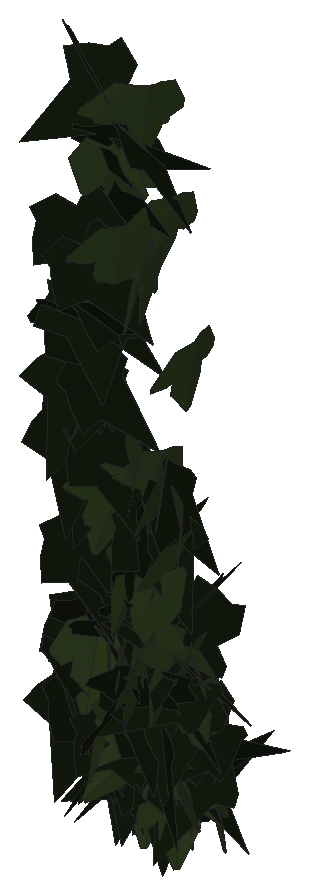
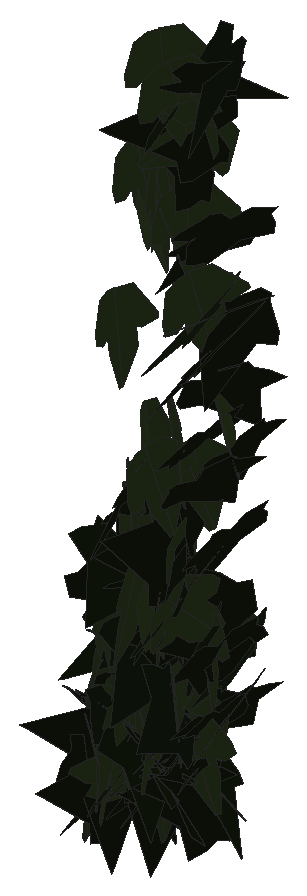
# SketchUp Ruby script. Lengths in inches.
U = 1.inch
M = Sketchup.active_model
def pt(a) = Geom::Point3d.new(a.map { |v| v * U })
def face(e, loops, mat)
  f = e.add_face(loops[0].map { |a| pt(a) })
  loops[1..].each { |l| e.add_face(l.map { |a| pt(a) }).erase! }
  f.material = f.back_material = mat if mat
  f
end
# faces: each face lists its corners as indices into pts; further lists are holes
def faces(e, pts, list, mat = nil) = list.each { |f| face(e, (f[0].is_a?(Array) ? f : [f]).map { |l| l.map { |i| pts[i] } }, mat) }
# xy, xz, yz: faces in a plane at the given z, y or x. An outline is a flat list of corners, or four numbers for a rectangle; further outlines are holes
def ring(l) = l.size == 4 ? [[l[0], l[1]], [l[2], l[1]], [l[2], l[3]], [l[0], l[3]]] : l.each_slice(2).to_a
def flat(e, list, mat, &to3) = list.each { |f| face(e, (f[0].is_a?(Array) ? f : [f]).map { |l| ring(l).map { |u, v| to3.(u, v) } }, mat) }
def xy(e, z, list, mat = nil) = flat(e, list, mat) { |x, y| [x, y, z] }
def xz(e, y, list, mat = nil) = flat(e, list, mat) { |x, z| [x, y, z] }
def yz(e, x, list, mat = nil) = flat(e, list, mat) { |y, z| [x, y, z] }
def lines(e, pts, list) = list.each { |a, b| e.add_line(pt(pts[a]), pt(pts[b])) }
# prism: a flat outline (further loops are holes) pulled along v
def prism(e, loops, v, mat = nil)
  f = face(e, loops, mat); d = Geom::Vector3d.new(v.map { |x| x * U })
  f.pushpull(f.normal.samedirection?(d) ? d.length : -d.length)
end
def box(e, o, s, mat = nil) = prism(e, [[o, [o[0] + s[0], o[1], o[2]], [o[0] + s[0], o[1] + s[1], o[2]], [o[0], o[1] + s[1], o[2]]]], [0, 0, s[2]], mat)
def at(x, y, z, deg = 0) = Geom::Transformation.translation(pt([x, y, z])) * Geom::Transformation.rotation(ORIGIN, Z_AXIS, deg.degrees)
def axes(o, x, y, z) = Geom::Transformation.new([*x, 0, *y, 0, *z, 0, *pt(o).to_a, 1])
def part(name) = M.definitions.add(name)
# library, detail: a bought-in or finely detailed component or shape, given as its bounding box
def library(name, o, s) = part(name).tap { |d| box(d.entities, o, s) }
def detail(e, o, s) = box(e.add_group.entities, o, s)
def put(e, d, t, mat = nil) = e.add_instance(d, t).tap { |i| i.material = mat if mat }
def group(e, t, mat = nil) = e.add_group.tap { |g| g.transformation = t; g.material = mat if mat }.entities
root = M.entities
M.materials.add("efeu1").color = [18, 25, 13]
M.materials.add("efeu2").color = [43, 57, 29]
c1 = part("ivyleaf_9")
p = [[1.54,2.16,1.25],[1.36,2.04,1.19],[-0.21,0.99,0.68],[-0.71,1.11,0.82],[-0.85,0.86,0.67],[-0.8,0.17,0.21],
  [-0.9,-0.01,0.1],[-0.67,-0.16,-0.02],[-0.08,-0.08,-0.05],[-0.03,-0.6,-0.4],[0.65,-0.88,-0.66],[0.83,-0.6,-0.49],
  [1.29,-0.42,-0.43],[1.8125,-0.07,-0.26],[1.21,0.44,0.15]]
faces(c1.entities,p,[[0,1,2,3,4,5,6,7,8,9,10,11,12,13,14]],"efeu1")
c2 = part("ivyleaf_10")
p = [[0,0.5,-0.03],[-0.0625,2.02,-0.43],[-0.19,2.01,-0.46],[-0.54,1.05,-0.29],[-0.52,0.625,-0.18],[-0.83,0.76,-0.28],
  [-1.16,0.64,-0.33],[-1.15,0.33,-0.24],[-0.77,-0.39,0.02],[-0.3,-0.51,0.16],[0.04,-0.48,0.23],[-0.02,2.01,-0.4375],
  [-0.06,2.01,-0.43],[0.04,-0.49,0.23],[0.67,-0.49,0.14],[1.38,0.36,-0.2],[1.375,0.51,-0.24],[0.81,0.65,-0.19],
  [0.62,0.59,-0.15],[0.6,1.09,-0.28],[0.5,1.23,-0.31]]
faces(c2.entities,p,[[0,1,2,3,4,5,6,7,8,9,10],[11,12,0,13,14,15,16,17,18,19,20]],"efeu2")
put(root,c1,axes([24.9,223.875,227.96],[-0.03734,-0.49581,0.05269],[-0.00909,-0.05215,-0.49719],[0.49852,-0.03809,-0.00512]))
put(root,c2,axes([25.2,224.25,223.83],[0.42311,-0.0185,-0.26577],[-0.23449,0.21088,-0.388],[0.12645,0.45297,0.16978]))
put(root,c1,axes([24.92,224.1,225.18],[0.01701,-0.48645,-0.11436],[-0.01724,0.11378,-0.48658],[0.49941,0.0205,-0.0129]))
put(root,c2,axes([25.09,223.83,228.52],[0.27311,-0.41851,0.01623],[0.00957,-0.01314,-0.49974],[0.41871,0.27328,0.00084]))
put(root,c1,axes([25.11,223.47,229.91],[0.3697,0.30061,-0.15152],[-0.13618,-0.07226,-0.47564],[-0.30786,0.39295,0.02845]))
put(root,c1,axes([24.91,223.53,224.96],[0.39664,-0.25422,-0.16747],[-0.09197,0.16213,-0.46396],[0.2902,0.39885,0.08185]))
put(root,c1,axes([24.92,223.74,224.14],[0.259,-0.41597,-0.09944],[-0.05405,0.08349,-0.49001],[0.42426,0.26458,-0.00172]))
put(root,c1,axes([25.13,223.63,233.63],[0.38485,-0.02875,-0.31791],[-0.3081,0.09677,-0.38172],[0.08348,0.4897,0.05677]))
put(root,c1,axes([25.16,223.85,228.86],[-0.29876,-0.4009,-0.00486],[0.00283,0.00395,-0.49998],[0.40092,-0.29877,-0.00009]))
put(root,c1,axes([25.07,224.11,222.95],[-0.05747,0.40596,-0.28617],[-0.06168,0.28001,0.40962],[0.49284,0.08239,0.0179]))
put(root,c1,axes([25.24,224.52,224.32],[0.07525,0.25877,0.42116],[0.02834,0.42306,-0.26499],[-0.49349,0.06375,0.049]))
put(root,c1,axes([24.93,224.39,224.26],[0.18953,-0.41983,-0.19448],[0.00009,0.2102,-0.45367],[0.46269,0.17194,0.07975]))
put(root,c1,axes([25.1,224.25,227.63],[-0.18158,-0.46064,0.06957],[0.00543,-0.07676,-0.49404],[0.46583,-0.17867,0.03288]))
put(root,c1,axes([25.08,223.86,224.08],[-0.14703,-0.46431,0.11314],[0.00838,-0.12086,-0.4851],[0.47782,-0.14075,0.04332]))
put(root,c2,axes([25.19,224.61,224.72],[0.23477,-0.41994,-0.13614],[-0.01582,0.1461,-0.47792],[0.44117,0.22871,0.05531]))
put(root,c1,axes([24.96,224.06,224.15],[0.18569,-0.40449,-0.22783],[-0.03218,0.23357,-0.44092],[0.46312,0.17841,0.06071]))
put(root,c1,axes([25.41,223.72,223.3],[-0.22871,0.44254,0.04299],[-0.01825,0.03896,-0.49815],[-0.44425,-0.22944,-0.00167]))
put(root,c1,axes([24.98,223.8,229.56],[0.17395,-0.46805,-0.02591],[0.02253,0.03595,-0.4982],[0.46822,0.17216,0.03359]))
put(root,c1,axes([25.02,223.74,231.22],[0.01891,-0.42163,-0.26809],[0.08632,0.267,-0.41383],[0.49213,-0.03063,0.08288]))
put(root,c2,axes([25.34,224.39,225.77],[0.14772,0.32658,-0.3486],[-0.20913,-0.28385,-0.35454],[-0.42947,0.25054,0.05274]))
put(root,c2,axes([25.31,223.83,225.2],[0.37751,-0.25512,-0.20592],[-0.08376,0.22856,-0.43674],[0.31697,0.36424,0.12983]))
put(root,c1,axes([25.11,223.63,226.6],[0.12625,-0.45515,-0.164],[-0.03084,0.16158,-0.47217],[0.48282,0.12933,0.01273]))
put(root,c1,axes([25.01,223.66,225.25],[0.32737,0.08964,0.36714],[0.34482,0.12797,-0.33871],[-0.15469,0.47496,0.02196]))
put(root,c2,axes([25.42,223.95,230.14],[-0.20271,-0.43927,0.12631],[-0.00107,-0.13771,-0.48066],[0.45706,-0.19514,0.05489]))
put(root,c1,axes([25.31,224.64,223.375],[-0.23606,-0.43533,-0.069],[0.04063,0.05645,-0.49514],[0.43889,-0.23938,0.00872]))
put(root,c1,axes([25.14,223.875,229.85],[-0.05658,-0.49678,0.00185],[0.1772,-0.02192,-0.46703],[0.46411,-0.0522,0.17854]))
put(root,c1,axes([25.6,223.9,233.13],[-0.39215,-0.1953,0.24099],[-0.18845,-0.15856,-0.43514],[0.2464,-0.4321,0.05075]))
put(root,c1,axes([25.16,223.87,229.99],[0.36504,-0.2859,-0.1871],[-0.06885,0.20663,-0.45007],[0.33467,0.35435,0.11149]))
put(root,c1,axes([25.13,224.14,223.58],[0.26347,-0.42121,0.05626],[0.02025,-0.05368,-0.4967],[0.42447,0.26401,-0.01123]))
put(root,c2,axes([25.41,223.625,225.24],[0.37271,0.32855,-0.05611],[-0.04662,-0.03196,-0.49679],[-0.33003,0.37555,0.00681]))
put(root,c1,axes([25.85,224.3125,222.99],[-0.20139,0.018,-0.45729],[-0.45662,-0.04133,0.19947],[-0.03062,0.49796,0.03309]))
put(root,c2,axes([25.5,224.51,223.46],[0.01115,-0.49259,-0.08504],[0.01777,0.0854,-0.49233],[0.49956,0.00796,0.01941]))
put(root,c1,axes([25.68,224.3,223.45],[-0.38287,0.25781,-0.19222],[0.09892,-0.18996,-0.45181],[-0.30598,-0.38399,0.09446]))
put(root,c2,axes([25.45,224.02,223.66],[-0.02991,-0.36564,-0.33972],[0.14889,0.3183,-0.35569],[0.47638,-0.12244,0.08984]))
put(root,c1,axes([25.3,224.12,226.02],[0.13597,-0.46864,0.10904],[0.03253,-0.1041,-0.48796],[0.48006,0.13979,0.00218]))
put(root,c1,axes([25.85,223.98,223.48],[-0.4524,0.1949,0.0857],[-0.08114,0.02825,-0.49256],[-0.19684,-0.45958,0.00606]))
put(root,c1,axes([25.45,224.46,223.46],[-0.11373,-0.48677,0.01121],[-0.00287,-0.01084,-0.49987],[0.48689,-0.11376,-0.00033]))
put(root,c1,axes([25.31,223.55,230.84],[0.14695,-0.3866,-0.28098],[0.0491,0.30462,-0.39344],[0.47539,0.08804,0.12748]))
put(root,c1,axes([25.78,224.52,223.6875],[-0.03757,0.48497,0.11574],[-0.07361,0.1094,-0.4823],[-0.49312,-0.05328,0.06318]))
put(root,c2,axes([25.6875,223.78,227.46],[-0.29374,-0.36021,0.18429],[-0.04949,-0.19404,-0.45815],[0.40158,-0.28739,0.07834]))
put(root,c2,axes([25.43,223.92,224.03],[-0.3174,-0.17678,-0.34352],[0.28878,0.18678,-0.36293],[0.25664,-0.42879,-0.01646]))
put(root,c2,axes([25.52,223.98,224.08],[0.07761,-0.32504,0.37192],[0.14468,-0.34501,-0.33171],[0.47227,0.15911,0.0405]))
put(root,c1,axes([25.39,223.47,229.16],[0.29346,-0.30224,-0.26932],[-0.07899,0.28349,-0.40422],[0.39704,0.27979,0.11864]))
put(root,c1,axes([25.38,223.8,228.01],[0.14786,-0.45519,-0.14471],[0.00546,0.15309,-0.47596],[0.47761,0.13917,0.05024]))
put(root,c1,axes([25.35,224.09,224.97],[0.09887,-0.34154,0.35153],[0.18408,-0.30648,-0.34955],[0.45425,0.19854,0.06514]))
put(root,c1,axes([25.73,224.26,223.29],[0.25444,0.39417,-0.17289],[-0.10681,-0.13673,-0.46893],[-0.41696,0.27556,0.01462]))
put(root,c1,axes([25.42,224.52,225.6875],[0.18051,-0.44663,0.13392],[0.06369,-0.11865,-0.48153],[0.46191,0.1909,0.01406]))
put(root,c1,axes([25.58,223.54,225.55],[0.3629,0.33503,0.07786],[0.06042,0.04933,-0.49388],[-0.33861,0.36786,-0.00468]))
put(root,c2,axes([25.77,223.76,225.33],[0.23914,-0.37135,-0.23432],[-0.04848,0.24286,-0.43436],[0.43642,0.23047,0.08015]))
put(root,c2,axes([25.8,223.64,231.13],[-0.22317,-0.44684,0.02305],[-0.00819,-0.02167,-0.49946],[0.44735,-0.22331,0.00235]))
put(root,c1,axes([25.82,223.28,224.31],[0.05577,0.40111,0.29326],[0.03897,0.29066,-0.40497],[-0.49535,0.06803,0.00115]))
put(root,c2,axes([25.52,223.58,232.38],[-0.21529,-0.20983,-0.39952],[0.36217,0.18374,-0.29167],[0.26922,-0.41498,0.07287]))
put(root,c1,axes([25.35,224.09,223.08],[0.34789,0.18804,-0.30596],[0.25695,0.16726,0.39497],[0.25089,-0.43205,0.01975]))
put(root,c2,axes([25.83,223.88,233.04],[-0.25752,-0.41224,0.11724],[-0.00377,-0.13459,-0.48153],[0.42857,-0.24889,0.06621]))
put(root,c1,axes([25.54,224.55,223.1875],[0.15715,-0.47347,0.03363],[0.00154,-0.03492,-0.49878],[0.47466,0.15687,-0.00951]))
put(root,c2,axes([25.85,224.29,227.59],[-0.08648,-0.47813,0.11795],[-0.00587,-0.11874,-0.48566],[0.49243,-0.08538,0.01493]))
put(root,c2,axes([25.83,224.48,223.51],[-0.21316,-0.43896,0.10898],[0.03655,-0.1368,-0.47953],[0.45081,-0.19647,0.09041]))
put(root,c2,axes([25.92,223.94,223.71],[-0.19839,-0.20561,0.41033],[-0.08658,-0.42223,-0.25343],[0.45072,-0.17161,0.13192]))
put(root,c1,axes([25.57,224.08,224],[0.32196,-0.36621,-0.1106],[-0.05263,0.10077,-0.4869],[0.37891,0.32517,0.02634]))
put(root,c1,axes([26.09,223.52,226.49],[-0.04756,0.06042,0.49405],[-0.21784,0.44372,-0.07524],[-0.44753,-0.22241,-0.01588]))
put(root,c1,axes([25.51,224.42,225.6],[0.09186,-0.22297,0.438],[0.18062,-0.39909,-0.24104],[0.4571,0.20251,0.00723]))
put(root,c1,axes([25.85,224.125,224.91],[0.22816,0.40693,0.17988],[-0.02422,0.21321,-0.45161],[-0.44425,0.19736,0.117]))
put(root,c2,axes([25.83,223.98,225.48],[0.1085,-0.45016,-0.18864],[0.03984,0.20077,-0.45619],[0.48646,0.08397,0.07944]))
put(root,c1,axes([25.43,223.59,232.34],[0.3556,-0.02951,0.35026],[0.35117,0.05138,-0.35219],[-0.01521,0.49648,0.05726]))
put(root,c2,axes([25.87,224.24,225.56],[0.08952,-0.48486,0.08304],[0.00652,-0.08323,-0.49298],[0.49188,0.08935,-0.00858]))
put(root,c2,axes([25.9,224.57,224.04],[-0.18975,-0.46213,-0.02067],[0.00196,0.02154,-0.49953],[0.46259,-0.18965,-0.00636]))
put(root,c2,axes([25.54,223.67,232.41],[-0.17671,0.03,-0.46677],[0.38946,-0.26688,-0.1646],[-0.25902,-0.42175,0.07095]))
put(root,c1,axes([25.64,223.81,224.05],[-0.02686,-0.36064,-0.34528],[0.12224,0.33051,-0.35471],[0.48408,-0.10347,0.07041]))
put(root,c1,axes([25.76,224.76,223.34],[-0.12304,-0.36494,0.31888],[0.00914,-0.33068,-0.37492],[0.48454,-0.08643,0.08804]))
put(root,c1,axes([25.79,223.875,226.08],[0.09471,0.00997,0.49085],[0.27163,0.41535,-0.06085],[-0.40896,0.27818,0.07325]))
put(root,c1,axes([25.75,224.53,223.1],[0.02255,-0.49806,0.03775],[0.00554,-0.03754,-0.49856],[0.49946,0.02291,0.00383]))
put(root,c2,axes([25.97,224.45,224.13],[-0.01772,-0.49937,-0.01766],[0.00029,0.01766,-0.49969],[0.49969,-0.01772,-0.00033]))
put(root,c2,axes([25.76,223.9,226.2],[-0.00787,-0.21693,0.45042],[0.27559,-0.37774,-0.17711],[0.41712,0.24547,0.12551]))
put(root,c1,axes([25.52,223.68,231.99],[0.18406,0.03692,-0.46342],[0.45658,0.07944,0.18767],[0.08748,-0.49227,-0.00448]))
put(root,c2,axes([25.99,223.67,227.97],[0.29328,-0.36902,-0.16678],[-0.05527,0.16752,-0.46785],[0.40116,0.29286,0.05747]))
put(root,c2,axes([25.82,224.14,223.23],[0.49218,0.04377,0.07641],[0.0761,0.00681,-0.49413],[-0.0443,0.49803,0.00004]))
put(root,c1,axes([25.72,224.03,224.37],[0.13049,-0.47307,0.0958],[0.04426,-0.0871,-0.49036],[0.48064,0.13646,0.01914]))
put(root,c2,axes([25.79,224.76,223.39],[0.16484,-0.22695,0.41391],[0.24549,-0.33325,-0.2805],[0.40319,0.2957,0.00156]))
put(root,c2,axes([25.99,224.47,225.86],[0.07345,-0.40503,-0.28383],[0.03219,0.29025,-0.40586],[0.49353,0.04135,0.06872]))
put(root,c2,axes([25.89,224.05,224.4],[0.22658,0.40585,0.18426],[0.02216,0.19619,-0.45937],[-0.44517,0.21633,0.07092]))
put(root,c1,axes([26.22,224.5625,224.07],[-0.23709,0.43648,-0.05726],[0.02856,-0.04964,-0.49671],[-0.43929,-0.2388,-0.00139]))
put(root,c2,axes([26.29,224.3,224.3],[-0.30848,0.23192,0.31789],[-0.34866,0.02617,-0.35742],[-0.18242,-0.44218,0.14558]))
put(root,c2,axes([25.82,223.97,224.46],[0.18768,0.23619,0.39874],[0.18706,0.35499,-0.29832],[-0.42401,0.26115,0.04489]))
put(root,c1,axes([26.16,224.55,223.74],[-0.47902,0.02512,-0.14111],[0.14111,-0.00356,-0.47966],[-0.0251,-0.49936,-0.00368]))
put(root,c2,axes([26.11,223.66,225.03],[0.17719,-0.46743,-0.01052],[-0.00215,0.01043,-0.49989],[0.46754,0.1772,0.00169]))
put(root,c1,axes([26.25,223.53,224.93],[0.17949,0.34432,-0.315],[-0.19318,-0.2524,-0.38597],[-0.42481,0.26026,0.04243]))
put(root,c2,axes([26.2,223.66,233.29],[-0.22055,-0.44856,0.01219],[0.00118,-0.01417,-0.4998],[0.44873,-0.22043,0.00731]))
put(root,c2,axes([26.03,224.64,223.26],[0.17975,0.41163,0.21965],[0.06333,0.21169,-0.44853],[-0.46226,0.18906,0.02397]))
put(root,c2,axes([26.11,223.7,230.96],[0.31646,-0.35837,0.14637],[0.08612,-0.11914,-0.4779],[0.37741,0.32768,-0.01369]))
put(root,c2,axes([26.42,224.16,224.45],[-0.41349,0.08739,0.26719],[-0.28111,-0.13168,-0.39197],[0.00186,-0.47437,0.15803]))
put(root,c1,axes([25.91,223.76,232.68],[0.34946,-0.35625,-0.03103],[-0.0145,0.02924,-0.49893],[0.3573,0.34962,0.0101]))
put(root,c1,axes([26.11,224.15,227.4],[0.27419,-0.28971,-0.30148],[-0.19003,0.23479,-0.39845],[0.37243,0.33308,0.01865]))
put(root,c1,axes([26.35,224.52,223.21],[0.03771,0.49504,-0.05926],[-0.00519,-0.05904,-0.49647],[-0.49855,0.03806,0.00068]))
put(root,c2,axes([26.31,224.25,224.4],[-0.29506,-0.4024,0.03187],[0.00529,-0.04332,-0.49809],[0.40362,-0.2936,0.02982]))
put(root,c2,axes([26.29,224.28,223.74],[-0.10247,-0.48935,0.00593],[0.03534,-0.01344,-0.49857],[0.48811,-0.10176,0.03734]))
put(root,c2,axes([26.45,224.67,223.12],[0.23041,-0.18263,0.40442],[-0.32683,0.2384,0.29385],[-0.30016,-0.39977,-0.00952]))
put(root,c2,axes([26.39,223.87,225.21],[-0.46764,-0.16341,0.06788],[-0.06908,-0.00801,-0.49514],[0.16291,-0.47247,-0.01508]))
put(root,c1,axes([26.05,224.6875,223.26],[0.33423,-0.34825,-0.13043],[-0.05853,0.12392,-0.48085],[0.36724,0.3367,0.04207]))
put(root,c2,axes([26.33,223.75,225.51],[0.10931,-0.4863,-0.03956],[-0.00696,0.03898,-0.49843],[0.48786,0.10951,0.00175]))
put(root,c1,axes([26.22,224.32,224.41],[-0.19938,-0.45086,-0.0835],[0.03216,0.07707,-0.49298],[0.4574,-0.20195,-0.00173]))
put(root,c2,axes([26.27,223.61,231.43],[0.12022,-0.47594,-0.09502],[0.07338,0.11459,-0.48113],[0.47975,0.10174,0.0974]))
put(root,c1,axes([26.09,223.95,226.96],[0.06779,-0.46263,-0.17715],[0.04136,0.18346,-0.46328],[0.49365,0.04816,0.06314]))
put(root,c2,axes([26.375,224.11,223.22],[-0.37716,0.3168,0.08597],[-0.08028,0.03795,-0.49205],[-0.31829,-0.38496,0.02223]))
put(root,c2,axes([26.33,223.77,231.05],[0.17112,-0.46595,0.06004],[0.01446,-0.05864,-0.49634],[0.46958,0.1716,-0.00659]))
put(root,c2,axes([26.36,224.0625,227.09],[0.32658,-0.32725,-0.19041],[-0.05086,0.21126,-0.45031],[0.37518,0.31349,0.1047]))
put(root,c1,axes([26.57,224.19,224.78],[-0.49293,-0.02248,0.08069],[-0.07123,-0.14093,-0.47441],[0.04407,-0.4792,0.13574]))
put(root,c1,axes([26.25,224.2,225.74],[-0.13433,-0.48128,0.01811],[-0.00497,-0.01742,-0.49967],[0.48159,-0.13442,-0.0001]))
put(root,c1,axes([26.22,224.5,222.78],[0.06064,0.09926,0.48628],[0.30623,0.37805,-0.11535],[-0.39057,0.31182,-0.01494]))
put(root,c2,axes([26.4,223.65,227.77],[0.14763,-0.44973,-0.16109],[-0.03401,0.15828,-0.47306],[0.4765,0.15063,0.01614]))
put(root,c2,axes([26.42,223.8,231.68],[-0.11875,-0.48143,0.06418],[-0.00029,-0.066,-0.49562],[0.48569,-0.11775,0.0154]))
put(root,c2,axes([26.29,224.1,223.1],[0.21415,0.45161,-0.01361],[-0.00451,-0.01293,-0.49981],[-0.4518,0.21419,-0.00147]))
put(root,c2,axes([26.34,224.72,223.05],[-0.36681,0.334,-0.06241],[0.03508,-0.05413,-0.49582],[-0.33797,-0.36812,0.01628]))
put(root,c1,axes([26.41,224.47,223.45],[-0.39697,-0.28725,-0.09951],[0.09517,0.03801,-0.48938],[0.28872,-0.40748,0.0245]))
put(root,c1,axes([26.12,223.98,223.78],[-0.11022,-0.00733,-0.48764],[0.48735,-0.02064,-0.10985],[-0.01852,-0.49952,0.01169]))
put(root,c1,axes([26.13,224.15,224.77],[0.34164,-0.36304,-0.03849],[-0.02414,0.03014,-0.49851],[0.36428,0.34248,0.00307]))
put(root,c2,axes([26.42,223.91,226.63],[0.06382,-0.4948,0.03318],[0.00835,-0.03238,-0.49888],[0.49584,0.06423,0.00413]))
put(root,c1,axes([26.14,224.17,225.13],[0.46069,-0.19419,-0.00773],[0.01946,0.06588,-0.49526],[0.19337,0.45602,0.06826]))
put(root,c2,axes([26.53,224.3,225.21],[-0.21079,0.3746,0.25543],[-0.14831,0.20922,-0.42922],[-0.42845,-0.25672,0.02291]))
put(root,c1,axes([26.07,224.41,223.54],[0.2992,-0.05248,0.39715],[0.40001,0.06607,-0.29262],[-0.02177,0.49283,0.08152]))
put(root,c1,axes([26.77,224.27,225.32],[-0.14481,-0.04913,0.47604],[-0.44768,-0.16189,-0.15289],[0.16916,-0.47051,0.0029]))
put(root,c1,axes([26.59,224.01,225.82],[0.11305,0.37496,0.31085],[-0.04232,0.32547,-0.3772],[-0.48521,0.05898,0.10533]))
put(root,c1,axes([26.69,224.55,223.98],[-0.4993,0.00624,-0.02574],[0.02431,-0.08468,-0.49218],[-0.0105,-0.49274,0.08426]))
put(root,c2,axes([26.46,223.92,225.3],[0.03131,-0.40433,0.29247],[0.13375,-0.27553,-0.39522],[0.48076,0.10298,0.0909]))
put(root,c2,axes([26.57,224.08,229.55],[-0.0157,-0.49331,-0.07997],[-0.00157,0.08006,-0.49355],[0.49975,-0.01525,-0.00407]))
put(root,c2,axes([26.55,224.36,225.23],[0.13229,-0.48051,-0.0401],[-0.00832,0.0393,-0.49838],[0.48211,0.13253,0.0024]))
put(root,c2,axes([26.24,223.58,225.875],[0.38267,-0.10884,-0.30285],[0.28821,-0.09343,0.39775],[-0.14317,-0.47898,-0.00877]))
